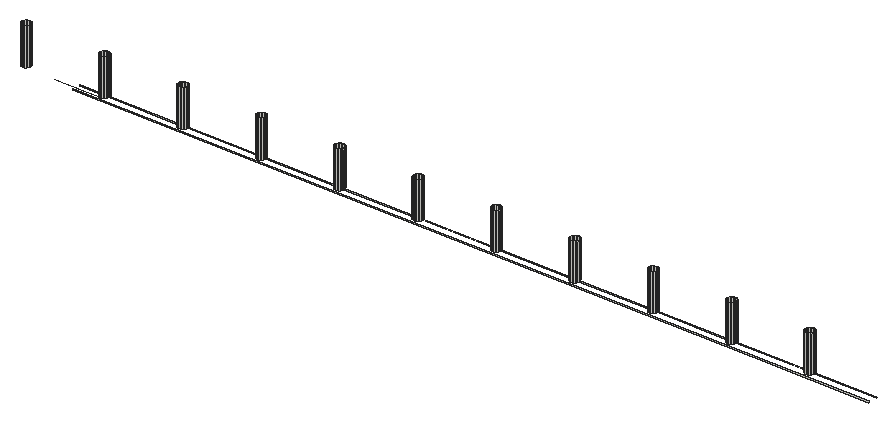
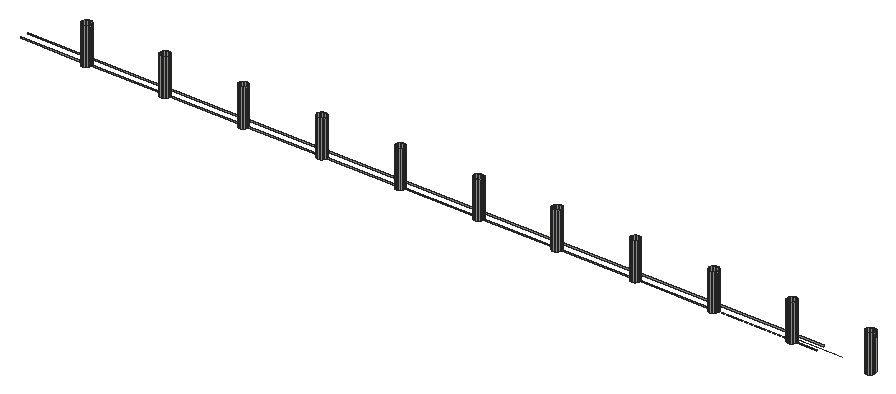
# SketchUp Ruby script. Lengths in inches.
U = 1.inch
M = Sketchup.active_model
def pt(a) = Geom::Point3d.new(a.map { |v| v * U })
def face(e, loops, mat)
  f = e.add_face(loops[0].map { |a| pt(a) })
  loops[1..].each { |l| e.add_face(l.map { |a| pt(a) }).erase! }
  f.material = f.back_material = mat if mat
  f
end
# faces: each face lists its corners as indices into pts; further lists are holes
def faces(e, pts, list, mat = nil) = list.each { |f| face(e, (f[0].is_a?(Array) ? f : [f]).map { |l| l.map { |i| pts[i] } }, mat) }
# xy, xz, yz: faces in a plane at the given z, y or x. An outline is a flat list of corners, or four numbers for a rectangle; further outlines are holes
def ring(l) = l.size == 4 ? [[l[0], l[1]], [l[2], l[1]], [l[2], l[3]], [l[0], l[3]]] : l.each_slice(2).to_a
def flat(e, list, mat, &to3) = list.each { |f| face(e, (f[0].is_a?(Array) ? f : [f]).map { |l| ring(l).map { |u, v| to3.(u, v) } }, mat) }
def xy(e, z, list, mat = nil) = flat(e, list, mat) { |x, y| [x, y, z] }
def xz(e, y, list, mat = nil) = flat(e, list, mat) { |x, z| [x, y, z] }
def yz(e, x, list, mat = nil) = flat(e, list, mat) { |y, z| [x, y, z] }
def lines(e, pts, list) = list.each { |a, b| e.add_line(pt(pts[a]), pt(pts[b])) }
# prism: a flat outline (further loops are holes) pulled along v
def prism(e, loops, v, mat = nil)
  f = face(e, loops, mat); d = Geom::Vector3d.new(v.map { |x| x * U })
  f.pushpull(f.normal.samedirection?(d) ? d.length : -d.length)
end
def box(e, o, s, mat = nil) = prism(e, [[o, [o[0] + s[0], o[1], o[2]], [o[0] + s[0], o[1] + s[1], o[2]], [o[0], o[1] + s[1], o[2]]]], [0, 0, s[2]], mat)
def at(x, y, z, deg = 0) = Geom::Transformation.translation(pt([x, y, z])) * Geom::Transformation.rotation(ORIGIN, Z_AXIS, deg.degrees)
def axes(o, x, y, z) = Geom::Transformation.new([*x, 0, *y, 0, *z, 0, *pt(o).to_a, 1])
def part(name) = M.definitions.add(name)
# library, detail: a bought-in or finely detailed component or shape, given as its bounding box
def library(name, o, s) = part(name).tap { |d| box(d.entities, o, s) }
def detail(e, o, s) = box(e.add_group.entities, o, s)
def put(e, d, t, mat = nil) = e.add_instance(d, t).tap { |i| i.material = mat if mat }
def group(e, t, mat = nil) = e.add_group.tap { |g| g.transformation = t; g.material = mat if mat }.entities
root = M.entities
xy(root,203.98,[[1390.64,569.58,1389.96,569.67,1389.32,569.93,1388.78,570.35,1388.36,570.89,1388.1,571.52,1388.02,572.14,1393.25,572.14,1393.17,571.52,1392.91,570.89,1392.49,570.35,1391.95,569.93,1391.32,569.67],[1388.02,572.14,1388.01,572.2,1393.26,572.2,1393.25,572.14],[938.64,572.2,938.73,572.88,938.99,573.52,939.41,574.06,939.95,574.48,940.58,574.74,941.26,574.83,941.94,574.74,942.57,574.48,943.12,574.06,943.53,573.52,943.8,572.88,943.89,572.2],[983.57,572.2,983.66,572.88,983.93,573.52,984.34,574.06,984.89,574.48,985.52,574.74,986.2,574.83,986.88,574.74,987.51,574.48,988.06,574.06,988.47,573.52,988.73,572.88,988.82,572.2],[1028.51,572.2,1028.6,572.88,1028.86,573.52,1029.28,574.06,1029.82,574.48,1030.46,574.74,1031.14,574.83,1031.82,574.74,1032.45,574.48,1032.99,574.06,1033.41,573.52,1033.67,572.88,1033.76,572.2],
  [1073.45,572.2,1073.54,572.88,1073.8,573.52,1074.22,574.06,1074.76,574.48,1075.39,574.74,1076.07,574.83,1076.75,574.74,1077.39,574.48,1077.93,574.06,1078.35,573.52,1078.61,572.88,1078.7,572.2],[1118.39,572.2,1118.48,572.88,1118.74,573.52,1119.16,574.06,1119.7,574.48,1120.33,574.74,1121.01,574.83,1121.69,574.74,1122.32,574.48,1122.87,574.06,1123.28,573.52,1123.55,572.88,1123.64,572.2],[1163.32,572.2,1163.41,572.88,1163.68,573.52,1164.09,574.06,1164.64,574.48,1165.27,574.74,1165.95,574.83,1166.63,574.74,1167.26,574.48,1167.81,574.06,1168.22,573.52,1168.48,572.88,1168.57,572.2],[1208.26,572.2,1208.35,572.88,1208.61,573.52,1209.03,574.06,1209.57,574.48,1210.21,574.74,1210.89,574.83,1211.57,574.74,1212.2,574.48,1212.74,574.06,1213.16,573.52,1213.42,572.88,1213.51,572.2],[1253.2,572.2,1253.29,572.88,1253.55,573.52,1253.97,574.06,1254.51,574.48,1255.14,574.74,1255.82,574.83,1256.5,574.74,1257.14,574.48,1257.68,574.06,1258.1,573.52,1258.36,572.88,1258.45,572.2],
  [1298.14,572.2,1298.23,572.88,1298.49,573.52,1298.91,574.06,1299.45,574.48,1300.08,574.74,1300.76,574.83,1301.44,574.74,1302.07,574.48,1302.62,574.06,1303.03,573.52,1303.3,572.88,1303.39,572.2],[1343.07,572.2,1343.16,572.88,1343.43,573.52,1343.84,574.06,1344.39,574.48,1345.02,574.74,1345.7,574.83,1346.38,574.74,1347.01,574.48,1347.56,574.06,1347.97,573.52,1348.23,572.88,1348.32,572.2],[1388.01,572.2,1388.1,572.88,1388.36,573.52,1388.78,574.06,1389.32,574.48,1389.96,574.74,1390.64,574.83,1391.32,574.74,1391.95,574.48,1392.49,574.06,1392.91,573.52,1393.17,572.88,1393.26,572.2]])
p = [[971.9,567.1,204.64],[971.9,567.02,203.98],[1361.8,567.02,203.98],[1428.71,567.02,203.98],[1428.71,567.1,204.64],[941.26,569.58,225.29],
  [940.58,569.67,225.29],[940.58,569.67,203.98],[941.26,569.58,203.98],[941.94,569.67,225.29],[941.94,569.67,203.98],[986.2,569.58,225.29],
  [985.52,569.67,225.29],[985.52,569.67,203.98],[986.2,569.58,203.98],[986.2,569.58,206.54],[986.88,569.67,225.29],[986.88,569.67,203.98],
  [1031.14,569.58,225.29],[1030.46,569.67,225.29],[1030.46,569.67,203.98],[1031.14,569.58,203.98],[1031.14,569.58,206.54],[1031.82,569.67,225.29],
  [1031.82,569.67,203.98],[1076.07,569.58,225.29],[1075.39,569.67,225.29],[1075.39,569.67,203.98],[1076.07,569.58,203.98],[1076.07,569.58,206.54],
  [1076.75,569.67,225.29],[1076.75,569.67,203.98],[1121.01,569.58,225.29],[1120.33,569.67,225.29],[1120.33,569.67,203.98],[1121.01,569.58,203.98],
  [1121.01,569.58,206.54],[1121.69,569.67,225.29],[1121.69,569.67,203.98],[1165.95,569.58,225.29],[1165.27,569.67,225.29],[1165.27,569.67,203.98],
  [1165.95,569.58,203.98],[1165.95,569.58,206.54],[1166.63,569.67,225.29],[1166.63,569.67,203.98],[1210.89,569.58,225.29],[1210.21,569.67,225.29],
  [1210.21,569.67,203.98],[1210.89,569.58,203.98],[1210.89,569.58,206.54],[1211.57,569.67,225.29],[1211.57,569.67,203.98],[1255.82,569.58,225.29],
  [1255.14,569.67,225.29],[1255.14,569.67,203.98],[1255.82,569.58,203.98],[1255.82,569.58,206.54],[1256.5,569.67,225.29],[1256.5,569.67,203.98],
  [1300.76,569.58,225.29],[1300.08,569.67,225.29],[1300.08,569.67,203.98],[1300.76,569.58,203.98],[1300.76,569.58,206.54],[1301.44,569.67,225.29],
  [1301.44,569.67,203.98],[1345.7,569.58,225.29],[1345.02,569.67,225.29],[1345.02,569.67,203.98],[1345.7,569.58,203.98],[1345.7,569.58,206.54],
  [1346.38,569.67,225.29],[1346.38,569.67,203.98],[1390.64,569.58,225.29],[1389.96,569.67,225.29],[1389.96,569.67,203.98],[1390.64,569.58,203.98],
  [1390.64,569.58,206.54],[1391.32,569.67,225.29],[1391.32,569.67,203.98],[939.95,569.93,225.29],[939.95,569.93,203.98],[942.57,569.93,225.29],
  [942.57,569.93,203.98],[984.89,569.93,225.29],[984.89,569.93,203.98],[987.51,569.93,225.29],[987.51,569.93,203.98],[1029.82,569.93,225.29],
  [1029.82,569.93,203.98],[1032.45,569.93,225.29],[1032.45,569.93,203.98],[1074.76,569.93,225.29],[1074.76,569.93,203.98],[1077.39,569.93,225.29],
  [1077.39,569.93,203.98],[1119.7,569.93,225.29],[1119.7,569.93,203.98],[1122.32,569.93,225.29],[1122.32,569.93,203.98],[1164.64,569.93,225.29],
  [1164.64,569.93,203.98],[1167.26,569.93,225.29],[1167.26,569.93,203.98],[1209.57,569.93,225.29],[1209.57,569.93,203.98],[1212.2,569.93,225.29],
  [1212.2,569.93,203.98],[1254.51,569.93,225.29],[1254.51,569.93,203.98],[1257.14,569.93,225.29],[1257.14,569.93,203.98],[1299.45,569.93,225.29],
  [1299.45,569.93,203.98],[1302.07,569.93,225.29],[1302.07,569.93,203.98],[1344.39,569.93,225.29],[1344.39,569.93,203.98],[1347.01,569.93,225.29],
  [1347.01,569.93,203.98],[1389.32,569.93,225.29],[1389.32,569.93,203.98],[1391.95,569.93,225.29],[1391.95,569.93,203.98],[939.41,570.35,225.29],
  [939.41,570.35,203.98],[943.12,570.35,225.29],[943.12,570.35,203.98],[984.34,570.35,225.29],[984.34,570.35,203.98],[988.06,570.35,225.29],
  [988.06,570.35,203.98],[1029.28,570.35,225.29],[1029.28,570.35,203.98],[1032.99,570.35,225.29],[1032.99,570.35,203.98],[1074.22,570.35,225.29],
  [1074.22,570.35,203.98],[1077.93,570.35,225.29],[1077.93,570.35,203.98],[1119.16,570.35,225.29],[1119.16,570.35,203.98],[1122.87,570.35,225.29],
  [1122.87,570.35,203.98],[1164.09,570.35,225.29],[1164.09,570.35,203.98],[1167.81,570.35,225.29],[1167.81,570.35,203.98],[1209.03,570.35,225.29],
  [1209.03,570.35,203.98],[1212.74,570.35,225.29],[1212.74,570.35,203.98],[1253.97,570.35,225.29],[1253.97,570.35,203.98],[1257.68,570.35,225.29],
  [1257.68,570.35,203.98],[1298.91,570.35,225.29],[1298.91,570.35,203.98],[1302.62,570.35,225.29],[1302.62,570.35,203.98],[1343.84,570.35,225.29],
  [1343.84,570.35,203.98],[1347.56,570.35,225.29],[1347.56,570.35,203.98],[1388.78,570.35,225.29],[1388.78,570.35,203.98],[1392.49,570.35,225.29],
  [1392.49,570.35,203.98],[938.99,570.89,225.29],[938.99,570.89,203.98],[943.53,570.89,225.29],[943.53,570.89,203.98],[983.93,570.89,225.29],
  [983.93,570.89,203.98],[988.47,570.89,225.29],[988.47,570.89,203.98],[1028.86,570.89,225.29],[1028.86,570.89,203.98],[1033.41,570.89,225.29],
  [1033.41,570.89,203.98],[1073.8,570.89,225.29],[1073.8,570.89,203.98],[1078.35,570.89,225.29],[1078.35,570.89,203.98],[1118.74,570.89,225.29],
  [1118.74,570.89,203.98],[1123.28,570.89,225.29],[1123.28,570.89,203.98],[1163.68,570.89,225.29],[1163.68,570.89,203.98],[1168.22,570.89,225.29],
  [1168.22,570.89,203.98],[1208.61,570.89,225.29],[1208.61,570.89,203.98],[1213.16,570.89,225.29],[1213.16,570.89,203.98],[1253.55,570.89,225.29],
  [1253.55,570.89,203.98],[1258.1,570.89,225.29],[1258.1,570.89,203.98],[1298.49,570.89,225.29],[1298.49,570.89,203.98],[1303.03,570.89,225.29],
  [1303.03,570.89,203.98],[1343.43,570.89,225.29],[1343.43,570.89,203.98],[1347.97,570.89,225.29],[1347.97,570.89,203.98],[1388.36,570.89,225.29],
  [1388.36,570.89,203.98],[1392.91,570.89,225.29],[1392.91,570.89,203.98],[938.73,571.52,225.29],[938.73,571.52,203.98],[943.8,571.52,225.29],
  [943.8,571.52,203.98],[983.66,571.52,225.29],[983.66,571.52,203.98],[988.73,571.52,225.29],[988.73,571.52,203.98],[1028.6,571.52,225.29],
  [1028.6,571.52,203.98],[1033.67,571.52,225.29],[1033.67,571.52,203.98],[1073.54,571.52,225.29],[1073.54,571.52,203.98],[1078.61,571.52,225.29],
  [1078.61,571.52,203.98],[1118.48,571.52,225.29],[1118.48,571.52,203.98],[1123.55,571.52,225.29],[1123.55,571.52,203.98],[1163.41,571.52,225.29],
  [1163.41,571.52,203.98],[1168.48,571.52,225.29],[1168.48,571.52,203.98],[1208.35,571.52,225.29],[1208.35,571.52,203.98],[1213.42,571.52,225.29],
  [1213.42,571.52,203.98],[1253.29,571.52,225.29],[1253.29,571.52,203.98],[1258.36,571.52,225.29],[1258.36,571.52,203.98],[1298.23,571.52,225.29],
  [1298.23,571.52,203.98],[1303.3,571.52,225.29],[1303.3,571.52,203.98],[1343.16,571.52,225.29],[1343.16,571.52,203.98],[1348.23,571.52,225.29],
  [1348.23,571.52,203.98],[1388.1,571.52,225.29],[1388.1,571.52,203.98],[1393.17,571.52,225.29],[1393.17,571.52,203.98],[938.64,572.2,225.29],
  [938.64,572.2,203.98],[943.89,572.2,225.29],[943.89,572.2,203.98],[983.57,572.2,225.29],[983.57,572.2,203.98],[983.58,572.14,203.98],
  [988.82,572.2,225.29],[988.82,572.14,203.98],[988.82,572.2,203.98],[1028.51,572.2,225.29],[1028.51,572.2,203.98],[1028.52,572.14,203.98],
  [1033.76,572.2,225.29],[1033.75,572.14,203.98],[1033.76,572.2,203.98],[1073.45,572.2,225.29],[1073.45,572.2,203.98],[1073.46,572.14,203.98],
  [1078.7,572.2,225.29],[1078.69,572.14,203.98],[1078.7,572.2,203.98],[1118.39,572.2,225.29],[1118.39,572.2,203.98],[1118.39,572.14,203.98],
  [1123.64,572.2,225.29],[1123.63,572.14,203.98],[1123.64,572.2,203.98],[1163.32,572.2,225.29],[1163.32,572.2,203.98],[1163.33,572.14,203.98],
  [1168.57,572.2,225.29],[1168.57,572.14,203.98],[1168.57,572.2,203.98],[1208.26,572.2,225.29],[1208.26,572.2,203.98],[1208.27,572.14,203.98],
  [1213.51,572.2,225.29],[1213.5,572.14,203.98],[1213.51,572.2,203.98],[1253.2,572.2,225.29],[1253.2,572.2,203.98],[1253.21,572.14,203.98],
  [1258.45,572.2,225.29],[1258.44,572.14,203.98],[1258.45,572.2,203.98],[1298.14,572.2,225.29],[1298.14,572.2,203.98],[1298.14,572.14,203.98],
  [1303.39,572.2,225.29],[1303.38,572.14,203.98],[1303.39,572.2,203.98],[1343.07,572.2,225.29],[1343.07,572.2,203.98],[1343.08,572.14,203.98],
  [1348.32,572.2,225.29],[1348.32,572.14,203.98],[1348.32,572.2,203.98],[1388.01,572.2,225.29],[1388.01,572.2,203.98],[1388.02,572.14,203.98],
  [1393.26,572.2,225.29],[1393.25,572.14,203.98],[1393.26,572.2,203.98],[971.9,572.14,203.98],[971.9,572.05,204.64],[1428.71,572.05,204.64],
  [1428.71,572.14,203.98],[938.73,572.88,225.29],[938.73,572.88,203.98],[943.8,572.88,225.29],[943.8,572.88,203.98],[983.66,572.88,225.29],
  [983.66,572.88,203.98],[988.73,572.88,225.29],[988.73,572.88,203.98],[1028.6,572.88,225.29],[1028.6,572.88,203.98],[1033.67,572.88,225.29],
  [1033.67,572.88,203.98],[1073.54,572.88,225.29],[1073.54,572.88,203.98],[1078.61,572.88,225.29],[1078.61,572.88,203.98],[1118.48,572.88,225.29],
  [1118.48,572.88,203.98],[1123.55,572.88,225.29],[1123.55,572.88,203.98],[1163.41,572.88,225.29],[1163.41,572.88,203.98],[1168.48,572.88,225.29],
  [1168.48,572.88,203.98],[1208.35,572.88,225.29],[1208.35,572.88,203.98],[1213.42,572.88,225.29],[1213.42,572.88,203.98],[1253.29,572.88,225.29],
  [1253.29,572.88,203.98],[1258.36,572.88,225.29],[1258.36,572.88,203.98],[1298.23,572.88,225.29],[1298.23,572.88,203.98],[1303.3,572.88,225.29],
  [1303.3,572.88,203.98],[1343.16,572.88,225.29],[1343.16,572.88,203.98],[1348.23,572.88,225.29],[1348.23,572.88,203.98],[1388.1,572.88,225.29],
  [1388.1,572.88,203.98],[1393.17,572.88,225.29],[1393.17,572.88,203.98],[938.99,573.52,225.29],[938.99,573.52,203.98],[943.53,573.52,225.29],
  [943.53,573.52,203.98],[983.93,573.52,225.29],[983.93,573.52,203.98],[988.47,573.52,225.29],[988.47,573.52,203.98],[1028.86,573.52,225.29],
  [1028.86,573.52,203.98],[1033.41,573.52,225.29],[1033.41,573.52,203.98],[1073.8,573.52,225.29],[1073.8,573.52,203.98],[1078.35,573.52,225.29],
  [1078.35,573.52,203.98],[1118.74,573.52,225.29],[1118.74,573.52,203.98],[1123.28,573.52,225.29],[1123.28,573.52,203.98],[1163.68,573.52,225.29],
  [1163.68,573.52,203.98],[1168.22,573.52,225.29],[1168.22,573.52,203.98],[1208.61,573.52,225.29],[1208.61,573.52,203.98],[1213.16,573.52,225.29],
  [1213.16,573.52,203.98],[1253.55,573.52,225.29],[1253.55,573.52,203.98],[1258.1,573.52,225.29],[1258.1,573.52,203.98],[1298.49,573.52,225.29],
  [1298.49,573.52,203.98],[1303.03,573.52,225.29],[1303.03,573.52,203.98],[1343.43,573.52,225.29],[1343.43,573.52,203.98],[1347.97,573.52,225.29],
  [1347.97,573.52,203.98],[1388.36,573.52,225.29],[1388.36,573.52,203.98],[1392.91,573.52,225.29],[1392.91,573.52,203.98],[939.41,574.06,225.29],
  [939.41,574.06,203.98],[943.12,574.06,225.29],[943.12,574.06,203.98],[984.34,574.06,225.29],[984.34,574.06,203.98],[988.06,574.06,225.29],
  [988.06,574.06,203.98],[1029.28,574.06,225.29],[1029.28,574.06,203.98],[1032.99,574.06,225.29],[1032.99,574.06,203.98],[1074.22,574.06,225.29],
  [1074.22,574.06,203.98],[1077.93,574.06,225.29],[1077.93,574.06,203.98],[1119.16,574.06,225.29],[1119.16,574.06,203.98],[1122.87,574.06,225.29],
  [1122.87,574.06,203.98],[1164.09,574.06,225.29],[1164.09,574.06,203.98],[1167.81,574.06,225.29],[1167.81,574.06,203.98],[1209.03,574.06,225.29],
  [1209.03,574.06,203.98],[1212.74,574.06,225.29],[1212.74,574.06,203.98],[1253.97,574.06,225.29],[1253.97,574.06,203.98],[1257.68,574.06,225.29],
  [1257.68,574.06,203.98],[1298.91,574.06,225.29],[1298.91,574.06,203.98],[1302.62,574.06,225.29],[1302.62,574.06,203.98],[1343.84,574.06,225.29],
  [1343.84,574.06,203.98],[1347.56,574.06,225.29],[1347.56,574.06,203.98],[1388.78,574.06,225.29],[1388.78,574.06,203.98],[1392.49,574.06,225.29],
  [1392.49,574.06,203.98],[939.95,574.48,225.29],[939.95,574.48,203.98],[942.57,574.48,225.29],[942.57,574.48,203.98],[984.89,574.48,225.29],
  [984.89,574.48,203.98],[987.51,574.48,225.29],[987.51,574.48,203.98],[1029.82,574.48,225.29],[1029.82,574.48,203.98],[1032.45,574.48,225.29],
  [1032.45,574.48,203.98],[1074.76,574.48,225.29],[1074.76,574.48,203.98],[1077.39,574.48,225.29],[1077.39,574.48,203.98],[1119.7,574.48,225.29],
  [1119.7,574.48,203.98],[1122.32,574.48,225.29],[1122.32,574.48,203.98],[1164.64,574.48,225.29],[1164.64,574.48,203.98],[1167.26,574.48,225.29],
  [1167.26,574.48,203.98],[1209.57,574.48,225.29],[1209.57,574.48,203.98],[1212.2,574.48,225.29],[1212.2,574.48,203.98],[1254.51,574.48,225.29],
  [1254.51,574.48,203.98],[1257.14,574.48,225.29],[1257.14,574.48,203.98],[1299.45,574.48,225.29],[1299.45,574.48,203.98],[1302.07,574.48,225.29],
  [1302.07,574.48,203.98],[1344.39,574.48,225.29],[1344.39,574.48,203.98],[1347.01,574.48,225.29],[1347.01,574.48,203.98],[1389.32,574.48,225.29],
  [1389.32,574.48,203.98],[1391.95,574.48,225.29],[1391.95,574.48,203.98],[940.58,574.74,225.29],[940.58,574.74,203.98],[941.94,574.74,225.29],
  [941.94,574.74,203.98],[985.52,574.74,225.29],[985.52,574.74,203.98],[986.88,574.74,225.29],[986.88,574.74,203.98],[1030.46,574.74,225.29],
  [1030.46,574.74,203.98],[1031.82,574.74,225.29],[1031.82,574.74,203.98],[1075.39,574.74,225.29],[1075.39,574.74,203.98],[1076.75,574.74,225.29],
  [1076.75,574.74,203.98],[1120.33,574.74,225.29],[1120.33,574.74,203.98],[1121.69,574.74,225.29],[1121.69,574.74,203.98],[1165.27,574.74,225.29],
  [1165.27,574.74,203.98],[1166.63,574.74,225.29],[1166.63,574.74,203.98],[1210.21,574.74,225.29],[1210.21,574.74,203.98],[1211.57,574.74,225.29],
  [1211.57,574.74,203.98],[1255.14,574.74,225.29],[1255.14,574.74,203.98],[1256.5,574.74,225.29],[1256.5,574.74,203.98],[1300.08,574.74,225.29],
  [1300.08,574.74,203.98],[1301.44,574.74,225.29],[1301.44,574.74,203.98],[1345.02,574.74,225.29],[1345.02,574.74,203.98],[1346.38,574.74,225.29],
  [1346.38,574.74,203.98],[1389.96,574.74,225.29],[1389.96,574.74,203.98],[1391.32,574.74,225.29],[1391.32,574.74,203.98],[941.26,574.83,225.29],
  [941.26,574.83,203.98],[986.2,574.83,225.29],[986.2,574.83,203.98],[1031.14,574.83,225.29],[1031.14,574.83,203.98],[1076.07,574.83,225.29],
  [1076.07,574.83,203.98],[1121.01,574.83,225.29],[1121.01,574.83,203.98],[1165.95,574.83,225.29],[1165.95,574.83,203.98],[1210.89,574.83,225.29],
  [1210.89,574.83,203.98],[1255.82,574.83,225.29],[1255.82,574.83,203.98],[1300.76,574.83,225.29],[1300.76,574.83,203.98],[1345.7,574.83,225.29],
  [1345.7,574.83,203.98],[1390.64,574.83,225.29],[1390.64,574.83,203.98],[971.9,569.58,203.98],[959.7,569.58,203.98]]
faces(root,p,[[0,1,2,3,4],[5,6,7,8],[9,5,8,10],[11,12,13,14,15],[16,11,15,14,17],[18,19,20,21,22],[23,18,22,21,24],[25,26,27,28,29],
  [30,25,29,28,31],[32,33,34,35,36],[37,32,36,35,38],[39,40,41,42,43],[44,39,43,42,45],[46,47,48,49,50],[51,46,50,49,52],[53,54,55,56,57],
  [58,53,57,56,59],[60,61,62,63,64],[65,60,64,63,66],[67,68,69,70,71],[72,67,71,70,73],[74,75,76,77,78],[79,74,78,77,80],[6,81,82,7],
  [83,9,10,84],[12,85,86,13],[87,16,17,88],[19,89,90,20],[91,23,24,92],[26,93,94,27],[95,30,31,96],[33,97,98,34],
  [99,37,38,100],[40,101,102,41],[103,44,45,104],[47,105,106,48],[107,51,52,108],[54,109,110,55],[111,58,59,112],[61,113,114,62],
  [115,65,66,116],[68,117,118,69],[119,72,73,120],[75,121,122,76],[123,79,80,124],[81,125,126,82],[127,83,84,128],[85,129,130,86],
  [131,87,88,132],[89,133,134,90],[135,91,92,136],[93,137,138,94],[139,95,96,140],[97,141,142,98],[143,99,100,144],[101,145,146,102],
  [147,103,104,148],[105,149,150,106],[151,107,108,152],[109,153,154,110],[155,111,112,156],[113,157,158,114],[159,115,116,160],[117,161,162,118],
  [163,119,120,164],[121,165,166,122],[167,123,124,168],[125,169,170,126],[171,127,128,172],[129,173,174,130],[175,131,132,176],[133,177,178,134],
  [179,135,136,180],[137,181,182,138],[183,139,140,184],[141,185,186,142],[187,143,144,188],[145,189,190,146],[191,147,148,192],[149,193,194,150],
  [195,151,152,196],[153,197,198,154],[199,155,156,200],[157,201,202,158],[203,159,160,204],[161,205,206,162],[207,163,164,208],[165,209,210,166],
  [211,167,168,212],[169,213,214,170],[215,171,172,216],[173,217,218,174],[219,175,176,220],[177,221,222,178],[223,179,180,224],[181,225,226,182],
  [227,183,184,228],[185,229,230,186],[231,187,188,232],[189,233,234,190],[235,191,192,236],[193,237,238,194],[239,195,196,240],[197,241,242,198],
  [243,199,200,244],[201,245,246,202],[247,203,204,248],[205,249,250,206],[251,207,208,252],[209,253,254,210],[255,211,212,256],[213,257,258,214],
  [259,215,216,260],[217,261,262,263,218],[264,219,220,265,266],[221,267,268,269,222],[270,223,224,271,272],[225,273,274,275,226],[276,227,228,277,278],[229,279,280,281,230],
  [282,231,232,283,284],[233,285,286,287,234],[288,235,236,289,290],[237,291,292,293,238],[294,239,240,295,296],[241,297,298,299,242],[300,243,244,301,302],[245,303,304,305,246],
  [306,247,248,307,308],[249,309,310,311,250],[312,251,252,313,314],[253,315,316,317,254],[318,255,256,319,320],[321,322,323,324,319,317,313,311,307,305,301,299,295,293,289,287,283,281,277,275,271,269,265,263],[257,325,326,258],[327,259,260,328],
  [261,329,330,262],[331,264,266,332],[267,333,334,268],[335,270,272,336],[273,337,338,274],[339,276,278,340],[279,341,342,280],[343,282,284,344],
  [285,345,346,286],[347,288,290,348],[291,349,350,292],[351,294,296,352],[297,353,354,298],[355,300,302,356],[303,357,358,304],[359,306,308,360],
  [309,361,362,310],[363,312,314,364],[315,365,366,316],[367,318,320,368],[325,369,370,326],[371,327,328,372],[329,373,374,330],[375,331,332,376],
  [333,377,378,334],[379,335,336,380],[337,381,382,338],[383,339,340,384],[341,385,386,342],[387,343,344,388],[345,389,390,346],[391,347,348,392],
  [349,393,394,350],[395,351,352,396],[353,397,398,354],[399,355,356,400],[357,401,402,358],[403,359,360,404],[361,405,406,362],[407,363,364,408],
  [365,409,410,366],[411,367,368,412],[369,413,414,370],[415,371,372,416],[373,417,418,374],[419,375,376,420],[377,421,422,378],[423,379,380,424],
  [381,425,426,382],[427,383,384,428],[385,429,430,386],[431,387,388,432],[389,433,434,390],[435,391,392,436],[393,437,438,394],[439,395,396,440],
  [397,441,442,398],[443,399,400,444],[401,445,446,402],[447,403,404,448],[405,449,450,406],[451,407,408,452],[409,453,454,410],[455,411,412,456],
  [413,457,458,414],[459,415,416,460],[417,461,462,418],[463,419,420,464],[421,465,466,422],[467,423,424,468],[425,469,470,426],[471,427,428,472],
  [429,473,474,430],[475,431,432,476],[433,477,478,434],[479,435,436,480],[437,481,482,438],[483,439,440,484],[441,485,486,442],[487,443,444,488],
  [445,489,490,446],[491,447,448,492],[449,493,494,450],[495,451,452,496],[453,497,498,454],[499,455,456,500],[457,501,502,458],[503,459,460,504],
  [461,505,506,462],[507,463,464,508],[465,509,510,466],[511,467,468,512],[469,513,514,470],[515,471,472,516],[473,517,518,474],[519,475,476,520],
  [477,521,522,478],[523,479,480,524],[481,525,526,482],[527,483,484,528],[485,529,530,486],[531,487,488,532],[489,533,534,490],[535,491,492,536],
  [493,537,538,494],[539,495,496,540],[497,541,542,498],[543,499,500,544],[501,545,546,502],[545,503,504,546],[505,547,548,506],[547,507,508,548],
  [509,549,550,510],[549,511,512,550],[513,551,552,514],[551,515,516,552],[517,553,554,518],[553,519,520,554],[521,555,556,522],[555,523,524,556],
  [525,557,558,526],[557,527,528,558],[529,559,560,530],[559,531,532,560],[533,561,562,534],[561,535,536,562],[537,563,564,538],[563,539,540,564],
  [541,565,566,542],[565,543,544,566]])
lines(root,p,[[14,567],[567,568]])
